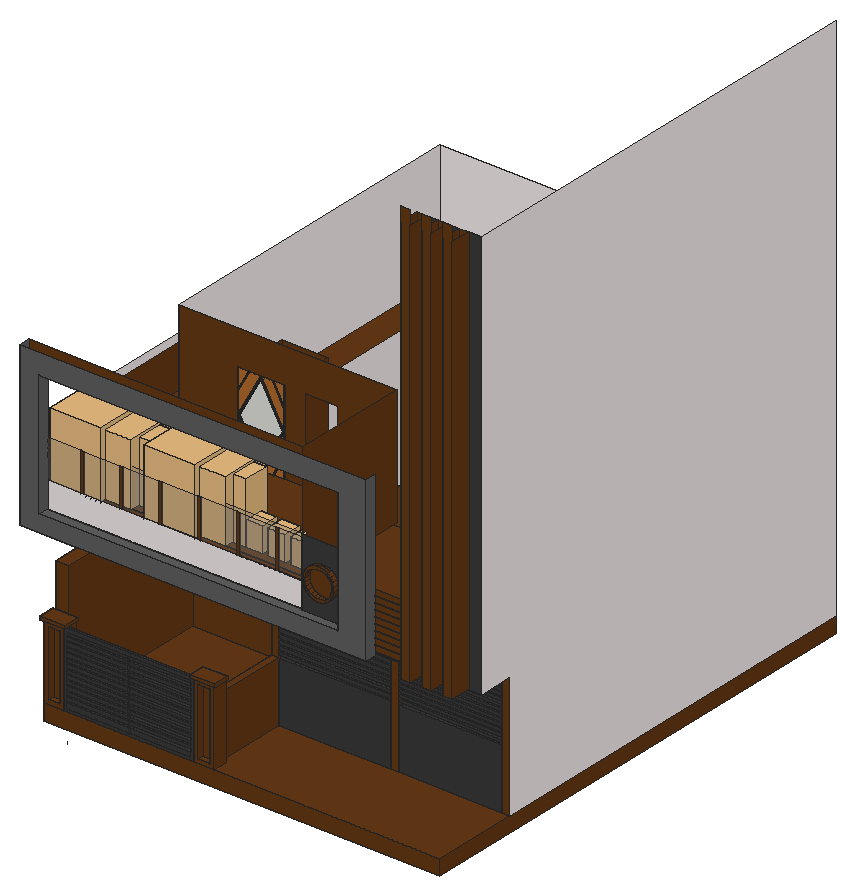
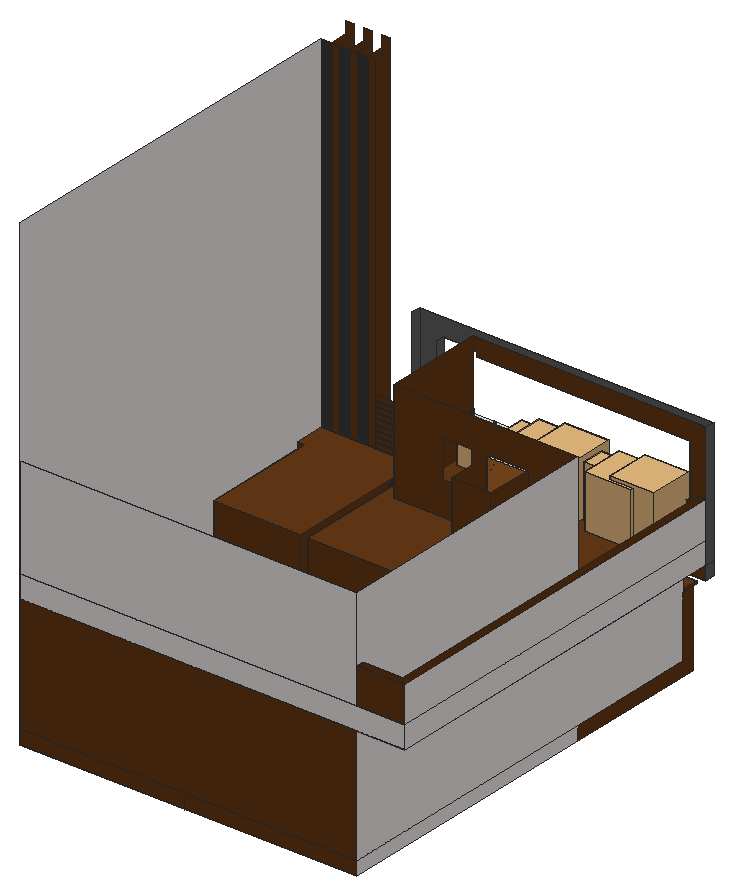
# SketchUp Ruby script. Lengths in inches.
U = 1.inch
M = Sketchup.active_model
def pt(a) = Geom::Point3d.new(a.map { |v| v * U })
def face(e, loops, mat)
  f = e.add_face(loops[0].map { |a| pt(a) })
  loops[1..].each { |l| e.add_face(l.map { |a| pt(a) }).erase! }
  f.material = f.back_material = mat if mat
  f
end
# faces: each face lists its corners as indices into pts; further lists are holes
def faces(e, pts, list, mat = nil) = list.each { |f| face(e, (f[0].is_a?(Array) ? f : [f]).map { |l| l.map { |i| pts[i] } }, mat) }
# xy, xz, yz: faces in a plane at the given z, y or x. An outline is a flat list of corners, or four numbers for a rectangle; further outlines are holes
def ring(l) = l.size == 4 ? [[l[0], l[1]], [l[2], l[1]], [l[2], l[3]], [l[0], l[3]]] : l.each_slice(2).to_a
def flat(e, list, mat, &to3) = list.each { |f| face(e, (f[0].is_a?(Array) ? f : [f]).map { |l| ring(l).map { |u, v| to3.(u, v) } }, mat) }
def xy(e, z, list, mat = nil) = flat(e, list, mat) { |x, y| [x, y, z] }
def xz(e, y, list, mat = nil) = flat(e, list, mat) { |x, z| [x, y, z] }
def yz(e, x, list, mat = nil) = flat(e, list, mat) { |y, z| [x, y, z] }
def lines(e, pts, list) = list.each { |a, b| e.add_line(pt(pts[a]), pt(pts[b])) }
# prism: a flat outline (further loops are holes) pulled along v
def prism(e, loops, v, mat = nil)
  f = face(e, loops, mat); d = Geom::Vector3d.new(v.map { |x| x * U })
  f.pushpull(f.normal.samedirection?(d) ? d.length : -d.length)
end
def box(e, o, s, mat = nil) = prism(e, [[o, [o[0] + s[0], o[1], o[2]], [o[0] + s[0], o[1] + s[1], o[2]], [o[0], o[1] + s[1], o[2]]]], [0, 0, s[2]], mat)
def at(x, y, z, deg = 0) = Geom::Transformation.translation(pt([x, y, z])) * Geom::Transformation.rotation(ORIGIN, Z_AXIS, deg.degrees)
def axes(o, x, y, z) = Geom::Transformation.new([*x, 0, *y, 0, *z, 0, *pt(o).to_a, 1])
def part(name) = M.definitions.add(name)
# library, detail: a bought-in or finely detailed component or shape, given as its bounding box
def library(name, o, s) = part(name).tap { |d| box(d.entities, o, s) }
def detail(e, o, s) = box(e.add_group.entities, o, s)
def put(e, d, t, mat = nil) = e.add_instance(d, t).tap { |i| i.material = mat if mat }
def group(e, t, mat = nil) = e.add_group.tap { |g| g.transformation = t; g.material = mat if mat }.entities
root = M.entities
M.materials.add("Generic").color = [102, 57, 22]
M.materials.add("Generic\#1").color = [96, 96, 96]
M.materials.add("Generic\#2").color = [59, 59, 59]
M.materials.add("Generic\#3").color = [243, 235, 235]
M.materials.add("[Color M07]").color = [58, 58, 58]
M.materials.add("[Color M08]").color = [30, 30, 30]
M.materials.add("[Translucent Glass Gray]").color = [128, 128, 128]
M.materials["[Translucent Glass Gray]"].alpha = 0.23
M.materials.add("[Wood Bamboo]").color = [177, 105, 43]
c1 = library("Raised potted plant",[1.65,0,0],[13.63,13.63,20.73])
c2 = library("Plant+2 (1)",[-9.13,-9.52,0],[51.76,51.77,66.88])
c3 = library("Group_2",[-1.28,-0.39,0],[21.22,20.51,48.44])
c4 = library("Flora+17",[-57.52,158.6,-38.64],[66.99,62.88,77.28])
c5 = part("Group\#4")
xy(c5.entities,0,[[10.55,0,10.55,0.4375,0,0.4375,0,3.4375,46.1875,3.4375,46.1875,0.4375,35.64,0.4375,35.64,0,34.64,0,34.64,0.4375,11.55,0.4375,11.55,0]])
xy(c5.entities,84.6875,[[11,0,11.55,0,11.55,0.4375,34.64,0.4375,34.64,0,35.1875,0,35.1875,0.4375,46.1875,0.4375,46.1875,3.4375,0,3.4375,0,0.4375,11,0.4375]])
xz(c5.entities,0,[[10.55,0,11.55,0,0,21.17,0,19.34],[[23.09,0,46.1875,42.34,23.09,84.6875,0,42.34],[23.09,2.875,1.57,42.34,23.09,81.8125,44.62,42.34]],[34.64,0,35.64,0,46.1875,19.34,46.1875,21.17],[0,63.52,11.55,84.6875,11,84.6875,0,64.52],[46.1875,63.52,46.1875,64.52,35.1875,84.6875,34.64,84.6875]],"[Color M08]")
xz(c5.entities,0.4375,[[23.09,2.875,44.62,42.34,23.09,81.8125,1.57,42.34]])
xz(c5.entities,0.4375,[[0,0,10.55,0,0,19.34],[11.55,0,23.09,0,0,42.34,0,21.17],[23.09,0,34.64,0,46.1875,21.17,46.1875,42.34],[35.64,0,46.1875,0,46.1875,19.34],[0,42.34,23.09,84.6875,11.55,84.6875,0,63.52],
  [46.1875,42.34,46.1875,63.52,34.64,84.6875,23.09,84.6875],[0,64.52,11,84.6875,0,84.6875],[46.1875,64.52,46.1875,84.6875,35.1875,84.6875]],"[Wood Bamboo]")
xz(c5.entities,3.4375,[[0,0,46.1875,84.6875]],"[Wood Bamboo]")
yz(c5.entities,0,[[0.4375,0,0.4375,19.34,0,19.34,0,21.17,0.4375,21.17,0.4375,63.52,0,63.52,0,64.52,0.4375,64.52,0.4375,84.6875,3.4375,84.6875,3.4375,0]],"[Wood Bamboo]")
yz(c5.entities,46.1875,[[0.4375,0,3.4375,0,3.4375,84.6875,0.4375,84.6875,0.4375,64.52,0,64.52,0,63.52,0.4375,63.52,0.4375,21.17,0,21.17,0,19.34,0.4375,19.34]],"[Wood Bamboo]")
p = [[0,0.4375,19.34],[10.55,0.4375,0],[10.55,0,0],[0,0,19.34],[0,0.4375,42.34],[23.09,0.4375,0],
  [23.09,0,0],[0,0,42.34],[11.55,0.4375,0],[0,0.4375,21.17],[0,0,21.17],[11.55,0,0],
  [46.1875,0.4375,42.34],[46.1875,0,42.34],[46.1875,0.4375,21.17],[34.64,0.4375,0],[34.64,0,0],[46.1875,0,21.17],
  [35.64,0.4375,0],[46.1875,0.4375,19.34],[46.1875,0,19.34],[35.64,0,0],[23.09,0.4375,2.875],[1.57,0.4375,42.34],
  [1.57,0,42.34],[23.09,0,2.875],[44.62,0.4375,42.34],[44.62,0,42.34],[23.09,0.4375,84.6875],[23.09,0,84.6875],
  [23.09,0.4375,81.8125],[23.09,0,81.8125],[0,0.4375,63.52],[11.55,0.4375,84.6875],[11.55,0,84.6875],[0,0,63.52],
  [34.64,0.4375,84.6875],[46.1875,0.4375,63.52],[46.1875,0,63.52],[34.64,0,84.6875],[11,0.4375,84.6875],[0,0.4375,64.52],
  [0,0,64.52],[11,0,84.6875],[46.1875,0.4375,64.52],[35.1875,0.4375,84.6875],[35.1875,0,84.6875],[46.1875,0,64.52]]
faces(c5.entities,p,[[0,1,2,3],[4,5,6,7],[8,9,10,11],[5,12,13,6],[14,15,16,17],[18,19,20,21],[22,23,24,25],[26,22,25,27],
  [28,4,7,29],[23,30,31,24],[12,28,29,13],[30,26,27,31],[32,33,34,35],[36,37,38,39],[40,41,42,43],[44,45,46,47]],"[Color M08]")
xy(root,-34.3125,[[288.56,2.3125,288.56,171.5,70.5625,171.5,70.5625,498.375,467.875,498.375,467.875,2.3125],[70.5625,2.3125,288.56,171.5]],"Generic")
xy(root,-18.375,[[70.5625,2.3125,90.75,16.625],[90.75,2.3125,220.74,2.3125,220.74,16.625,228.93,16.625,228.93,171.5,84.25,171.5,84.25,16.625,90.75,16.625],[220.74,2.3125,240.93,2.3125,240.93,16.625,236.43,16.625,236.43,171.5,228.93,171.5,228.93,16.625,220.74,16.625],[240.93,2.3125,467.875,2.3125,467.875,89.8125,459.25,89.8125,459.25,223.75,356.47,223.75,356.47,89.8125,347.84,89.8125,347.84,223.75,236.43,223.75,236.43,16.625,240.93,16.625],[70.5625,16.625,84.25,16.625,84.25,171.5,236.43,171.5,236.43,223.75,347.84,223.75,347.84,89.8125,356.47,89.8125,356.47,223.75,459.25,223.75,459.25,89.8125,467.875,89.8125,467.875,498.375,70.5625,498.375]],"Generic")
xy(root,-14.21,[[224.91,2.3125,236.77,8.6875]],"Generic")
xy(root,-13.73,[[75.21,2.3125,86.1,8.6875]],"Generic")
xy(root,42.625,[[228.93,16.625,236.43,89.8125]],"Generic")
xy(root,52.54,[[75.21,2.3125,86.1,8.6875]],"Generic")
xy(root,53.02,[[224.91,2.3125,236.77,8.6875]],"Generic")
xy(root,57.1875,[[68.25,0,68.25,16.625,70.5625,16.625,70.5625,2.3125,93.0625,2.3125,93.0625,0],[218.43,0,218.43,2.3125,240.93,2.3125,240.93,16.625,243.24,16.625,243.24,0],[90.75,2.3125,93.0625,16.625],[218.43,2.3125,220.74,16.625],[220.74,2.3125,240.93,16.625]],"Generic")
xy(root,60.375,[[68.25,0,93.0625,16.625],[218.43,0,243.24,16.625]],"Generic")
xy(root,103.625,[[70.5625,16.625,84.25,43.5625],[70.5625,43.5625,84.25,54.375]],"Generic")
xy(root,103.625,[[13.1875,43.5625,70.5625,54.375],[84.25,43.5625,360.31,54.375]],"Generic\#1")
xy(root,106.1875,[[228.93,54.375,228.93,89.8125,236.43,89.8125,236.43,223.75,347.84,223.75,347.84,89.8125,356.47,89.8125,356.47,223.75,459.25,223.75,459.25,89.8125,467.875,89.8125,467.875,54.375]],"Generic")
xy(root,106.625,[[403,33.625,412.5,54.375],[424.1875,33.625,433.6875,54.375],[445.375,33.625,454.875,54.375],[360.31,54.375,403,54.68]],"Generic")
xy(root,107.625,[[360.31,54.375,403,54.68]],"Generic")
xy(root,112.9375,[[360.31,54.375,403,54.68]],"Generic")
xy(root,113.9375,[[360.31,54.375,403,54.68]],"Generic")
xy(root,119.25,[[360.31,54.375,403,54.68]],"Generic")
xy(root,120,[[288.56,53.375,331.74,54.375],[[13.1875,54.375,70.5625,171.5],[28.32,79.86,59.77,99.3]],[84.25,54.375,228.93,171.5],[28.32,79.86,59.77,99.3],[13.1875,171.5,70.5625,498.375]],"Generic")
xy(root,120,[[32.25,43.5625,331.74,43.5625,331.74,53.375,288.56,53.375,288.56,54.375,32.25,54.375]],"Generic\#1")
xy(root,120.25,[[360.31,54.375,403,54.68]],"Generic")
xy(root,125.5625,[[360.31,54.375,403,54.68]],"Generic")
xy(root,126.5625,[[360.31,54.375,403,54.68]],"Generic")
xy(root,131.875,[[360.31,54.375,403,54.68]],"Generic")
xy(root,132.875,[[360.31,54.375,403,54.68]],"Generic")
xy(root,138.1875,[[360.31,54.375,403,54.68]],"Generic")
xy(root,139.1875,[[360.31,54.375,403,54.68]],"Generic")
xy(root,144.5,[[360.31,54.375,403,54.68]],"Generic")
xy(root,145.5,[[360.31,54.375,403,54.68]],"Generic")
xy(root,145.75,[[13.1875,54.375,13.1875,498.375,70.5625,498.375,70.5625,489.875,22.72,489.875,22.72,54.375],[22.72,54.375,22.72,489.875,70.5625,489.875,70.5625,171.5,129.97,171.5,129.97,226.25,176.16,226.25,176.16,171.5,288.56,171.5,288.56,59.625,32.25,59.625,32.25,54.375],[32.25,54.375,288.56,59.625]],"Generic")
xy(root,150.8125,[[360.31,54.375,403,54.68]],"Generic")
xy(root,151.8125,[[360.31,54.375,403,54.68]],"Generic")
xy(root,157.125,[[360.31,54.375,403,54.68]],"Generic")
xy(root,158.125,[[360.31,54.375,403,54.68]],"Generic")
xz(root,0,[[68.25,57.1875,93.0625,60.375],[218.43,57.1875,243.24,60.375]],"Generic")
xz(root,2.3125,[[70.5625,-34.3125,467.875,-18.375],[[70.5625,-18.375,90.75,57.1875],[75.21,-13.73,86.1,52.54]],[[220.74,-18.375,240.93,57.1875],[224.91,-14.21,236.77,53.02]]],"Generic")
xz(root,8.6875,[[224.91,-14.21,236.77,53.02],[75.21,-13.73,86.1,52.54]],"Generic")
xz(root,16.625,[[70.5625,-18.375,84.25,57.1875],[84.25,-18.375,90.75,57.1875],[220.74,-18.375,220.74,57.1875,240.93,57.1875,240.93,-18.375,236.43,-18.375,236.43,42.625,228.93,42.625,228.93,-18.375],[68.25,57.1875,70.5625,60.375],[70.5625,57.1875,84.25,60.375],
  [84.25,57.1875,93.0625,60.375],[218.43,57.1875,243.24,60.375],[70.5625,60.375,84.25,103.625]],"Generic")
xz(root,33.625,[[403,106.625,412.5,531.8125],[424.1875,106.625,433.6875,531.8125],[445.375,106.625,454.875,531.8125]],"Generic")
xz(root,43.5625,[[[13.1875,103.625,360.31,265.75],[32.25,120,331.74,245.11]]],"Generic\#1")
xz(root,47.75,[[[307.6875,136.43,311.86,136.55,315.86,137.76,319.41,139.96,322.27,143,324.25,146.68,325.2,150.75,325.07,154.93,323.87,158.92,321.67,162.47,318.625,165.34,314.94,167.31,310.88,168.27,306.7,168.14,302.7,166.93,299.15,164.73,296.29,161.6875,294.32,158.01,293.36,153.94,293.49,149.77,294.7,145.77,296.9,142.22,299.94,139.36,303.62,137.38],[307.93,138.8,304.47,139.61,301.34,141.3,298.75,143.73,296.875,146.75,295.85,150.15,295.74,153.7,296.55,157.16,298.23,160.29,300.67,162.88,303.6875,164.75,307.09,165.78,310.64,165.89,314.1,165.08,317.23,163.4,319.82,160.96,321.6875,157.94,322.72,154.54,322.83,150.99,322.01,147.53,320.33,144.4,317.9,141.81,314.88,139.9375,311.48,138.91]]],"Generic")
xz(root,53.375,[[307.93,138.8,311.48,138.91,314.88,139.9375,317.9,141.81,320.33,144.4,322.01,147.53,322.83,150.99,322.72,154.54,321.6875,157.94,319.82,160.96,317.23,163.4,314.1,165.08,310.64,165.89,307.09,165.78,303.6875,164.75,300.67,162.88,298.23,160.29,296.55,157.16,295.74,153.7,295.85,150.15,296.875,146.75,298.75,143.73,301.34,141.3,304.47,139.61]],"Generic")
xz(root,53.375,[[[288.56,120,331.74,188.375],[307.6875,136.43,303.62,137.38,299.94,139.36,296.9,142.22,294.7,145.77,293.49,149.77,293.36,153.94,294.32,158.01,296.29,161.6875,299.15,164.73,302.7,166.93,306.7,168.14,310.88,168.27,314.94,167.31,318.625,165.34,321.67,162.47,323.87,158.92,325.07,154.93,325.2,150.75,324.25,146.68,322.27,143,319.41,139.96,315.86,137.76,311.86,136.55]]],"Generic\#2")
xz(root,54.375,[[13.1875,103.625,70.5625,120],[70.5625,103.625,84.25,120],[84.25,103.625,228.93,120],[228.93,103.625,360.31,106.1875],[228.93,106.1875,360.31,106.625],
  [228.93,106.625,360.31,107.625],[403,106.625,412.5,517.125],[424.1875,106.625,433.6875,517.125],[445.375,106.625,454.875,517.125],[228.93,107.625,360.31,112.9375],
  [360.31,107.625,403,112.9375],[228.93,112.9375,360.31,113.9375],[228.93,113.9375,360.31,119.25],[360.31,113.9375,403,119.25],[228.93,119.25,360.31,119.25,360.31,120.25,331.74,120.25,331.74,120,228.93,120],
  [13.1875,120,32.25,145.75],[288.56,120,331.74,120.25],[331.74,120.25,360.31,125.5625],[360.31,120.25,403,125.5625],[288.56,125.5625,331.74,126.5625],
  [331.74,125.5625,360.31,126.5625],[331.74,126.5625,360.31,131.875],[360.31,126.5625,403,131.875],[288.56,131.875,331.74,132.875],[331.74,131.875,360.31,132.875],
  [331.74,132.875,360.31,138.1875],[360.31,132.875,403,138.1875],[288.56,138.1875,331.74,139.1875],[331.74,138.1875,360.31,139.1875],[331.74,139.1875,360.31,144.5],
  [360.31,139.1875,403,144.5],[288.56,144.5,331.74,145.5],[331.74,144.5,360.31,145.5],[331.74,145.5,360.31,150.8125],[360.31,145.5,403,150.8125],
  [13.1875,145.75,22.72,188.56],[22.72,145.75,22.72,188.56,13.1875,188.56,13.1875,265.75,288.56,265.75,288.56,250.86,284.06,250.86,284.06,245.11,32.25,245.11,32.25,145.75],[66,145.75,69,184.5625],[105.0625,145.75,108.0625,184.5625],[144.125,145.75,147.125,184.5625],
  [183.1875,145.75,186.1875,184.5625],[222.25,145.75,225.25,184.5625],[261.3125,145.75,264.3125,184.5625],[288.56,150.8125,331.74,151.8125],[331.74,150.8125,360.31,151.8125],
  [331.74,151.8125,360.31,157.125],[360.31,151.8125,403,157.125],[288.56,157.125,331.74,158.125],[331.74,157.125,360.31,158.125],[331.74,158.125,360.31,163.4375],
  [360.31,158.125,403,163.4375]],"Generic")
xz(root,54.375,[[360.31,106.1875,467.875,106.1875,467.875,517.125,454.875,517.125,454.875,106.625,445.375,106.625,445.375,517.125,433.6875,517.125,433.6875,106.625,424.1875,106.625,424.1875,517.125,412.5,517.125,412.5,106.625,360.31,106.625]],"Generic\#2")
xz(root,54.375,[[32.25,120,288.56,145.75]],"Generic\#3")
xz(root,54.375,[[32.25,145.75,66,184.5625],[69,145.75,105.0625,184.5625],[108.0625,145.75,144.125,184.5625],[147.125,145.75,183.1875,184.5625],[186.1875,145.75,222.25,184.5625],
  [225.25,145.75,261.3125,184.5625],[264.3125,145.75,288.56,184.5625]],"[Translucent Glass Gray]")
xz(root,54.68,[[360.31,106.625,403,107.625],[360.31,112.9375,403,113.9375],[360.31,119.25,403,120.25],[360.31,125.5625,403,126.5625],[360.31,131.875,403,132.875],
  [360.31,138.1875,403,139.1875],[360.31,144.5,403,145.5],[360.31,150.8125,403,151.8125],[360.31,157.125,403,158.125]],"Generic")
xz(root,59.625,[[32.25,145.75,288.56,184.5625]],"[Translucent Glass Gray]")
xz(root,89.8125,[[347.84,-18.375,356.47,106.1875],[459.25,-18.375,467.875,106.1875],[228.93,42.625,236.43,106.1875]],"Generic")
xz(root,171.5,[[84.25,-18.375,228.93,120],[[70.5625,145.75,129.97,145.75,129.97,230.4375,176.16,230.4375,176.16,145.75,288.56,145.75,288.56,265.75,70.5625,265.75],[196.46,185.5625,230.03,230.4375]]],"Generic")
xz(root,223.75,[[236.43,-18.375,347.84,106.1875],[356.47,-18.375,459.25,106.1875]],"Generic")
xz(root,226.25,[[129.97,145.75,176.16,230.4375]],"Generic")
xz(root,489.875,[[22.72,145.75,70.5625,188.56]],"Generic")
xz(root,498.375,[[70.5625,-34.3125,467.875,-18.375],[70.5625,-18.375,467.875,120],[13.1875,145.75,70.5625,188.56]],"Generic")
xz(root,498.375,[[13.1875,120,467.875,145.75],[70.5625,145.75,467.875,265.75]],"Generic\#3")
yz(root,13.1875,[[43.5625,103.625,54.375,120],[43.5625,120,54.375,265.75]],"Generic\#1")
yz(root,13.1875,[[54.375,120,498.375,145.75],[54.375,145.75,498.375,188.56]],"Generic\#3")
yz(root,22.72,[[54.375,145.75,489.875,188.56]],"Generic")
yz(root,32.25,[[54.375,145.75,59.625,184.5625]],"Generic")
yz(root,32.25,[[43.5625,120,54.375,245.11]],"Generic\#1")
yz(root,68.25,[[0,57.1875,16.625,60.375]],"Generic")
yz(root,70.5625,[[2.3125,-34.3125,171.5,-18.375],[2.3125,-18.375,16.625,57.1875]],"Generic")
yz(root,70.5625,[[171.5,-34.3125,498.375,-18.375],[16.625,-18.375,16.625,103.625,54.375,103.625,54.375,120,498.375,120,498.375,-18.375],[171.5,145.75,171.5,265.75,498.375,265.75,498.375,188.56,489.875,188.56,489.875,145.75]],"Generic\#3")
yz(root,75.21,[[2.3125,-13.73,8.6875,52.54]],"Generic")
yz(root,84.25,[[16.625,-18.375,171.5,-18.375,171.5,120,54.375,120,54.375,103.625,16.625,103.625]],"Generic")
yz(root,86.1,[[2.3125,-13.73,8.6875,52.54]],"Generic")
yz(root,90.75,[[2.3125,-18.375,16.625,57.1875]],"Generic")
yz(root,93.0625,[[0,57.1875,16.625,60.375]],"Generic")
yz(root,129.97,[[171.5,145.75,226.25,230.4375]],"Generic")
yz(root,176.16,[[171.5,145.75,226.25,230.4375]],"Generic")
yz(root,218.43,[[0,57.1875,16.625,60.375]],"Generic")
yz(root,220.74,[[2.3125,-18.375,16.625,57.1875]],"Generic")
yz(root,224.91,[[2.3125,-14.21,8.6875,53.02]],"Generic")
yz(root,228.93,[[16.625,-18.375,16.625,42.625,89.8125,42.625,89.8125,106.1875,54.375,106.1875,54.375,120,171.5,120,171.5,-18.375]],"Generic")
yz(root,236.43,[[16.625,-18.375,223.75,-18.375,223.75,106.1875,89.8125,106.1875,89.8125,42.625,16.625,42.625]],"Generic")
yz(root,236.77,[[2.3125,-14.21,8.6875,53.02]],"Generic")
yz(root,240.93,[[2.3125,-18.375,16.625,57.1875]],"Generic")
yz(root,243.24,[[0,57.1875,16.625,60.375]],"Generic")
yz(root,288.56,[[53.375,120,54.375,145.75],[53.375,145.75,54.375,184.5625],[54.375,145.75,59.625,184.5625],[59.625,145.75,59.625,188.375,54.375,188.375,54.375,265.75,171.5,265.75,171.5,145.75]],"Generic")
yz(root,331.74,[[53.375,120,54.375,188.375]],"Generic")
yz(root,331.74,[[43.5625,120,43.5625,245.11,54.375,245.11,54.375,188.375,53.375,188.375,53.375,120]],"Generic\#1")
yz(root,347.84,[[89.8125,-18.375,223.75,106.1875]],"Generic")
yz(root,356.47,[[89.8125,-18.375,223.75,106.1875]],"Generic")
yz(root,360.31,[[54.375,106.625,54.68,107.625],[54.375,112.9375,54.68,113.9375],[54.375,119.25,54.68,120.25],[54.375,125.5625,54.68,126.5625],[54.375,131.875,54.68,132.875],
  [54.375,138.1875,54.68,139.1875],[54.375,144.5,54.68,145.5],[54.375,150.8125,54.68,151.8125],[54.375,157.125,54.68,158.125]],"Generic")
yz(root,360.31,[[43.5625,103.625,54.375,265.75]],"Generic\#1")
yz(root,403,[[33.625,106.625,54.375,517.125],[54.375,106.625,54.68,107.625],[54.375,112.9375,54.68,113.9375],[54.375,119.25,54.68,120.25],[54.375,125.5625,54.68,126.5625],
  [54.375,131.875,54.68,132.875],[54.375,138.1875,54.68,139.1875],[54.375,144.5,54.68,145.5],[54.375,150.8125,54.68,151.8125],[54.375,157.125,54.68,158.125]],"Generic")
yz(root,412.5,[[33.625,106.625,54.375,517.125]],"Generic")
yz(root,424.1875,[[33.625,106.625,54.375,517.125]],"Generic")
yz(root,433.6875,[[33.625,106.625,54.375,517.125]],"Generic")
yz(root,445.375,[[33.625,106.625,54.375,517.125]],"Generic")
yz(root,454.875,[[33.625,106.625,54.375,517.125]],"Generic")
yz(root,459.25,[[89.8125,-18.375,223.75,106.1875]],"Generic")
yz(root,467.875,[[2.3125,-34.3125,498.375,-18.375]],"Generic")
yz(root,467.875,[[89.8125,-18.375,498.375,-18.375,498.375,517.125,54.375,517.125,54.375,106.1875,89.8125,106.1875]],"Generic\#3")
p = [[303.62,53.375,137.38],[307.6875,53.375,136.43],[307.6875,47.75,136.43],[303.62,47.75,137.38],[311.86,53.375,136.55],[311.86,47.75,136.55],
  [315.86,53.375,137.76],[315.86,47.75,137.76],[299.94,53.375,139.36],[299.94,47.75,139.36],[319.41,53.375,139.96],[319.41,47.75,139.96],
  [307.93,53.375,138.8],[304.47,53.375,139.61],[304.47,47.75,139.61],[307.93,47.75,138.8],[311.48,53.375,138.91],[311.48,47.75,138.91],
  [314.88,53.375,139.9375],[314.88,47.75,139.9375],[296.9,53.375,142.22],[296.9,47.75,142.22],[301.34,53.375,141.3],[301.34,47.75,141.3],
  [317.9,53.375,141.81],[317.9,47.75,141.81],[322.27,53.375,143],[322.27,47.75,143],[298.75,53.375,143.73],[298.75,47.75,143.73],
  [320.33,53.375,144.4],[320.33,47.75,144.4],[294.7,53.375,145.77],[294.7,47.75,145.77],[324.25,53.375,146.68],[324.25,47.75,146.68],
  [296.875,53.375,146.75],[296.875,47.75,146.75],[322.01,53.375,147.53],[322.01,47.75,147.53],[293.49,53.375,149.77],[293.49,47.75,149.77],
  [295.85,53.375,150.15],[295.85,47.75,150.15],[325.2,53.375,150.75],[325.2,47.75,150.75],[322.83,53.375,150.99],[322.83,47.75,150.99],
  [293.36,53.375,153.94],[293.36,47.75,153.94],[295.74,53.375,153.7],[295.74,47.75,153.7],[325.07,53.375,154.93],[325.07,47.75,154.93],
  [322.72,53.375,154.54],[322.72,47.75,154.54],[296.55,53.375,157.16],[296.55,47.75,157.16],[294.32,53.375,158.01],[294.32,47.75,158.01],
  [321.6875,53.375,157.94],[321.6875,47.75,157.94],[323.87,53.375,158.92],[323.87,47.75,158.92],[298.23,53.375,160.29],[298.23,47.75,160.29],
  [319.82,53.375,160.96],[319.82,47.75,160.96],[296.29,53.375,161.6875],[296.29,47.75,161.6875],[321.67,53.375,162.47],[321.67,47.75,162.47],
  [300.67,53.375,162.88],[300.67,47.75,162.88],[317.23,53.375,163.4],[317.23,47.75,163.4],[299.15,53.375,164.73],[299.15,47.75,164.73],
  [318.625,53.375,165.34],[318.625,47.75,165.34],[303.6875,53.375,164.75],[303.6875,47.75,164.75],[288.56,171.5,-18.375],[288.56,171.5,-34.3125]]
faces(root,p,[[0,1,2,3],[1,4,5,2],[4,6,7,5],[8,0,3,9],[6,10,11,7],[12,13,14,15],[16,12,15,17],[18,16,17,19],
  [20,8,9,21],[13,22,23,14],[24,18,19,25],[10,26,27,11],[22,28,29,23],[30,24,25,31],[32,20,21,33],[26,34,35,27],
  [28,36,37,29],[38,30,31,39],[40,32,33,41],[36,42,43,37],[34,44,45,35],[46,38,39,47],[48,40,41,49],[42,50,51,43],
  [44,52,53,45],[54,46,47,55],[50,56,57,51],[58,48,49,59],[60,54,55,61],[52,62,63,53],[56,64,65,57],[66,60,61,67],
  [68,58,59,69],[62,70,71,63],[64,72,73,65],[74,66,67,75],[76,68,69,77],[70,78,79,71],[72,80,81,73]],"Generic")
lines(root,p,[[82,83]])
g1 = group(root,at(90.75,2.3125,-47.375))
xy(g1,29,[[0,0,129.99,3]],"[Color M07]")
xy(g1,37.5625,[[2.8125,0,64,3],[66,0,127.18,3]],"[Color M07]")
xy(g1,39.5,[[2.8125,0,64,3],[66,0,127.18,3]],"[Color M07]")
xy(g1,42.5,[[2.8125,0,64,3],[66,0,127.18,3]],"[Color M07]")
xy(g1,44.4375,[[2.8125,0,64,3],[66,0,127.18,3]],"[Color M07]")
xy(g1,47.4375,[[2.8125,0,64,3],[66,0,127.18,3]],"[Color M07]")
xy(g1,49.375,[[2.8125,0,64,3],[66,0,127.18,3]],"[Color M07]")
xy(g1,52.375,[[2.8125,0,64,3],[66,0,127.18,3]],"[Color M07]")
xy(g1,54.3125,[[2.8125,0,64,3],[66,0,127.18,3]],"[Color M07]")
xy(g1,57.3125,[[2.8125,0,64,3],[66,0,127.18,3]],"[Color M07]")
xy(g1,59.25,[[2.8125,0,64,3],[66,0,127.18,3]],"[Color M07]")
xy(g1,62.25,[[2.8125,0,64,3],[66,0,127.18,3]],"[Color M07]")
xy(g1,64.1875,[[2.8125,0,64,3],[66,0,127.18,3]],"[Color M07]")
xy(g1,67.1875,[[2.8125,0,64,3],[66,0,127.18,3]],"[Color M07]")
xy(g1,69.125,[[2.8125,0,64,3],[66,0,127.18,3]],"[Color M07]")
xy(g1,72.125,[[2.8125,0,64,3],[66,0,127.18,3]],"[Color M07]")
xy(g1,74.0625,[[2.8125,0,64,3],[66,0,127.18,3]],"[Color M07]")
xy(g1,77.0625,[[2.8125,0,64,3],[66,0,127.18,3]],"[Color M07]")
xy(g1,79,[[2.8125,0,64,3],[66,0,127.18,3]],"[Color M07]")
xy(g1,82,[[2.8125,0,64,3],[66,0,127.18,3]],"[Color M07]")
xy(g1,83.9375,[[2.8125,0,64,3],[66,0,127.18,3]],"[Color M07]")
xy(g1,86.9375,[[2.8125,0,64,3],[66,0,127.18,3]],"[Color M07]")
xy(g1,88.875,[[2.8125,0,64,3],[66,0,127.18,3]],"[Color M07]")
xy(g1,91.875,[[2.8125,0,64,3],[66,0,127.18,3]],"[Color M07]")
xy(g1,93.8125,[[2.8125,0,64,3],[66,0,127.18,3]],"[Color M07]")
xy(g1,96.8125,[[2.8125,0,64,3],[66,0,127.18,3]],"[Color M07]")
xy(g1,98.75,[[2.8125,0,64,3],[66,0,127.18,3]],"[Color M07]")
xy(g1,104.5625,[[0,0,2.3125,3],[2.3125,0,127.68,3],[127.68,0,129.99,3]],"[Color M07]")
xz(g1,0,[[[0,29,129.99,104.5625],[2.8125,31.82,127.18,101.75]],[2.8125,31.82,64,37.5625],[64,31.82,66,101.75],[66,31.82,127.18,37.5625],[2.8125,39.5,64,42.5],
  [66,39.5,127.18,42.5],[2.8125,44.4375,64,47.4375],[66,44.4375,127.18,47.4375],[2.8125,49.375,64,52.375],[66,49.375,127.18,52.375],
  [2.8125,54.3125,64,57.3125],[66,54.3125,127.18,57.3125],[2.8125,59.25,64,62.25],[66,59.25,127.18,62.25],[2.8125,64.1875,64,67.1875],
  [66,64.1875,127.18,67.1875],[2.8125,69.125,64,72.125],[66,69.125,127.18,72.125],[2.8125,74.0625,64,77.0625],[66,74.0625,127.18,77.0625],
  [2.8125,79,64,82],[66,79,127.18,82],[2.8125,83.9375,64,86.9375],[66,83.9375,127.18,86.9375],[2.8125,88.875,64,91.875],
  [66,88.875,127.18,91.875],[2.8125,93.8125,64,96.8125],[66,93.8125,127.18,96.8125],[2.8125,98.75,64,101.75],[66,98.75,127.18,101.75]],"[Color M07]")
xz(g1,3,[[[0,29,129.99,104.5625],[66,37.5625,127.18,39.5],[66,42.5,127.18,44.4375],[66,47.4375,127.18,49.375],[66,52.375,127.18,54.3125],[66,57.3125,127.18,59.25],[66,62.25,127.18,64.1875],[66,67.1875,127.18,69.125],[66,72.125,127.18,74.0625],[66,77.0625,127.18,79],[66,82,127.18,83.9375],[66,86.9375,127.18,88.875],[66,91.875,127.18,93.8125],[66,96.8125,127.18,98.75],[2.8125,91.875,64,93.8125],[2.8125,86.9375,64,88.875],[2.8125,82,64,83.9375],[2.8125,77.0625,64,79],[2.8125,72.125,64,74.0625],[2.8125,62.25,64,64.1875],[2.8125,67.1875,64,69.125],[2.8125,57.3125,64,59.25],[2.8125,52.375,64,54.3125],[2.8125,47.4375,64,49.375],[2.8125,42.5,64,44.4375],[2.8125,37.5625,64,39.5],[2.8125,96.8125,64,98.75]]],"[Color M07]")
yz(g1,0,[[0,29,3,104.5625]],"[Color M07]")
yz(g1,2.8125,[[0,37.5625,3,39.5],[0,42.5,3,44.4375],[0,47.4375,3,49.375],[0,52.375,3,54.3125],[0,57.3125,3,59.25],
  [0,62.25,3,64.1875],[0,67.1875,3,69.125],[0,72.125,3,74.0625],[0,77.0625,3,79],[0,82,3,83.9375],
  [0,86.9375,3,88.875],[0,91.875,3,93.8125],[0,96.8125,3,98.75]],"[Color M07]")
yz(g1,64,[[0,37.5625,3,39.5],[0,42.5,3,44.4375],[0,47.4375,3,49.375],[0,52.375,3,54.3125],[0,57.3125,3,59.25],
  [0,62.25,3,64.1875],[0,67.1875,3,69.125],[0,72.125,3,74.0625],[0,77.0625,3,79],[0,82,3,83.9375],
  [0,86.9375,3,88.875],[0,91.875,3,93.8125],[0,96.8125,3,98.75]],"[Color M07]")
yz(g1,66,[[0,37.5625,3,39.5],[0,42.5,3,44.4375],[0,47.4375,3,49.375],[0,52.375,3,54.3125],[0,57.3125,3,59.25],
  [0,62.25,3,64.1875],[0,67.1875,3,69.125],[0,72.125,3,74.0625],[0,77.0625,3,79],[0,82,3,83.9375],
  [0,86.9375,3,88.875],[0,91.875,3,93.8125],[0,96.8125,3,98.75]],"[Color M07]")
yz(g1,127.18,[[0,37.5625,3,39.5],[0,42.5,3,44.4375],[0,47.4375,3,49.375],[0,52.375,3,54.3125],[0,57.3125,3,59.25],
  [0,62.25,3,64.1875],[0,67.1875,3,69.125],[0,72.125,3,74.0625],[0,77.0625,3,79],[0,82,3,83.9375],
  [0,86.9375,3,88.875],[0,91.875,3,93.8125],[0,96.8125,3,98.75]],"[Color M07]")
yz(g1,129.99,[[0,29,3,104.5625]],"[Color M07]")
p = [[181.375,499.0625,29],[181.375,499.0625,13.0625],[2.8125,0,3],[2.8125,0,0]]
lines(g1,p,[[0,1],[2,3]])
g2 = group(root,at(236.43,89.8125,-18.375))
box(g2,[120.03,0,86.125],[102.79,3,2.625],"[Color M07]")
box(g2,[120.03,0,90.75],[102.79,3,2.625],"[Color M07]")
box(g2,[120.03,0,76.875],[102.79,3,2.625],"[Color M07]")
box(g2,[120.03,0,81.5],[102.79,3,2.625],"[Color M07]")
box(g2,[120.03,0,100],[102.79,3,2.625],"[Color M07]")
box(g2,[120.03,0,67.625],[102.79,3,2.625],"[Color M07]")
box(g2,[120.03,0,63],[102.79,3,2.625],"[Color M07]")
box(g2,[120.03,0,72.25],[102.79,3,2.625],"[Color M07]")
box(g2,[120.03,0,95.375],[102.79,3,2.625],"[Color M07]")
box(g2,[120.03,0,109.25],[102.79,3,2.625],"[Color M07]")
box(g2,[120.03,0,104.625],[102.79,3,2.625],"[Color M07]")
box(g2,[120.03,0,113.875],[102.79,3,2.625],"[Color M07]")
box(g2,[0,0,120.75],[111.41,3,1.25],"[Color M07]")
box(g2,[0,0,115.5],[111.41,3,3.25],"[Color M07]")
box(g2,[0,0,110.25],[111.41,3,3.25],"[Color M07]")
box(g2,[0,0,105],[111.41,3,3.25],"[Color M07]")
box(g2,[0,0,99.75],[111.41,3,3.25],"[Color M07]")
box(g2,[0,0,94.5],[111.41,3,3.25],"[Color M07]")
box(g2,[0,0,89.25],[111.41,3,3.25],"[Color M07]")
box(g2,[0,0,78.75],[111.41,3,3.25],"[Color M07]")
box(g2,[0,0,73.5],[111.41,3,3.25],"[Color M07]")
box(g2,[0,0,84],[111.41,3,3.25],"[Color M07]")
box(g2,[120.03,0,118.5],[102.79,3,3.5],"[Color M07]")
box(g2,[0,0,0],[111.41,3,61],"[Color M07]")
box(g2,[120.03,0,0],[102.79,3,61],"[Color M07]")
box(g2,[0,0,68.25],[111.41,3,3.25],"[Color M07]")
box(g2,[0,0,63],[111.41,3,3.25],"[Color M07]")
p = [[0,3,63],[0,3,61],[0,3,120.75],[0,3,118.75],[222.82,3,72.25],[222.82,3,70.25],
  [222.82,3,100],[222.82,3,98],[222.82,3,67.625],[222.82,3,65.625],[222.82,3,104.625],[222.82,3,102.625],
  [222.82,3,76.875],[222.82,3,74.875],[222.82,3,81.5],[222.82,3,79.5],[0,3,94.5],[0,3,92.5],
  [0,3,84],[0,3,82],[222.82,3,90.75],[222.82,3,88.75],[0,3,89.25],[0,3,87.25],
  [0,3,115.5],[0,3,113.5],[0,3,105],[0,3,103],[222.82,3,118.5],[222.82,3,116.5],
  [0,3,99.75],[0,3,97.75],[0,3,110.25],[0,3,108.25],[0,3,78.75],[0,3,76.75],
  [0,3,68.25],[0,3,66.25],[222.82,3,113.875],[222.82,3,111.875],[222.82,3,95.375],[222.82,3,93.375],
  [0,3,73.5],[0,3,71.5],[222.82,3,63],[222.82,3,61],[222.82,3,86.125],[222.82,3,84.125],
  [222.82,3,109.25],[222.82,3,107.25]]
lines(g2,p,[[0,1],[2,3],[4,5],[6,7],[8,9],[10,11],[12,13],[14,15],[16,17],[18,19],[20,21],[22,23],
  [24,25],[26,27],[28,29],[30,31],[32,33],[34,35],[36,37],[38,39],[40,41],[42,43],[44,45],[46,47],
  [48,49]])
put(root,c1,axes([27.65,68.41,143.54],[1.31,0,0],[0,1.31,0],[0,0,1.31]))
put(root,c1,axes([122.09,68.41,143.54],[1.31,0,0],[0,1.31,0],[0,0,1.31]))
put(root,c1,axes([216.59,68.41,143.54],[1.31,0,0],[0,1.31,0],[0,0,1.31]))
put(root,c1,axes([239.59,68.41,143.54],[1.31,0,0],[0,1.31,0],[0,0,1.31]))
put(root,c1,axes([262.59,68.41,143.54],[1.31,0,0],[0,1.31,0],[0,0,1.31]))
put(root,c2,at(43.25,63.9,144.7))
put(root,c2,at(137.68,63.9,144.7))
put(root,c3,axes([100.88,68.54,145.75],[1.26,0,0],[0,1.26,0],[0,0,1.26]))
put(root,c3,axes([195.32,68.54,145.75],[1.26,0,0],[0,1.26,0],[0,0,1.26]))
put(root,c4,axes([104.85,-69.4,177.05],[0.81,0,0],[0,0.81,0],[0,0,0.81]))
put(root,c4,axes([199.29,-69.4,177.05],[0.81,0,0],[0,0.81,0],[0,0,0.81]))
put(root,c5,at(129.97,171.0625,145.75))
